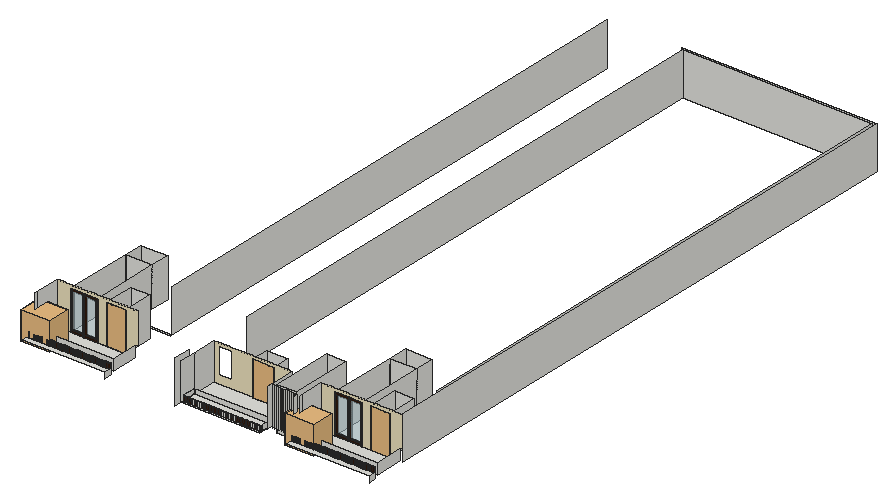
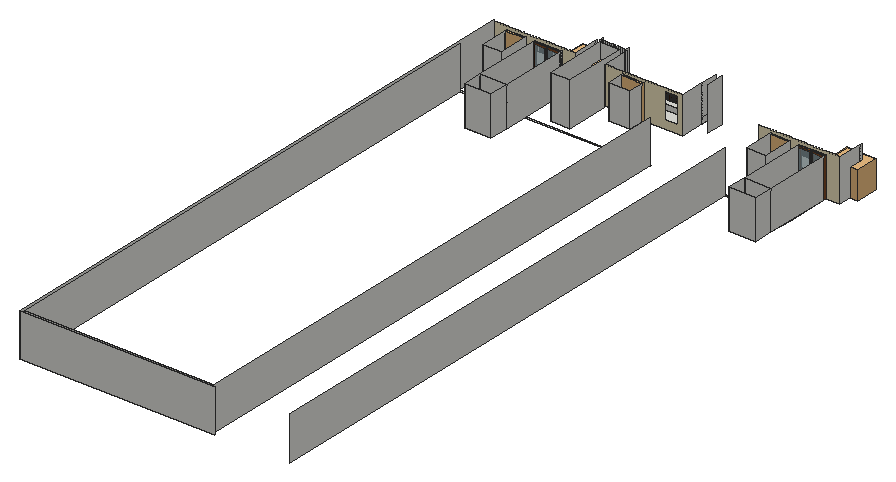
# SketchUp Ruby script. Lengths in inches.
U = 1.inch
M = Sketchup.active_model
def pt(a) = Geom::Point3d.new(a.map { |v| v * U })
def face(e, loops, mat)
  f = e.add_face(loops[0].map { |a| pt(a) })
  loops[1..].each { |l| e.add_face(l.map { |a| pt(a) }).erase! }
  f.material = f.back_material = mat if mat
  f
end
# faces: each face lists its corners as indices into pts; further lists are holes
def faces(e, pts, list, mat = nil) = list.each { |f| face(e, (f[0].is_a?(Array) ? f : [f]).map { |l| l.map { |i| pts[i] } }, mat) }
# xy, xz, yz: faces in a plane at the given z, y or x. An outline is a flat list of corners, or four numbers for a rectangle; further outlines are holes
def ring(l) = l.size == 4 ? [[l[0], l[1]], [l[2], l[1]], [l[2], l[3]], [l[0], l[3]]] : l.each_slice(2).to_a
def flat(e, list, mat, &to3) = list.each { |f| face(e, (f[0].is_a?(Array) ? f : [f]).map { |l| ring(l).map { |u, v| to3.(u, v) } }, mat) }
def xy(e, z, list, mat = nil) = flat(e, list, mat) { |x, y| [x, y, z] }
def xz(e, y, list, mat = nil) = flat(e, list, mat) { |x, z| [x, y, z] }
def yz(e, x, list, mat = nil) = flat(e, list, mat) { |y, z| [x, y, z] }
def lines(e, pts, list) = list.each { |a, b| e.add_line(pt(pts[a]), pt(pts[b])) }
# prism: a flat outline (further loops are holes) pulled along v
def prism(e, loops, v, mat = nil)
  f = face(e, loops, mat); d = Geom::Vector3d.new(v.map { |x| x * U })
  f.pushpull(f.normal.samedirection?(d) ? d.length : -d.length)
end
def box(e, o, s, mat = nil) = prism(e, [[o, [o[0] + s[0], o[1], o[2]], [o[0] + s[0], o[1] + s[1], o[2]], [o[0], o[1] + s[1], o[2]]]], [0, 0, s[2]], mat)
def at(x, y, z, deg = 0) = Geom::Transformation.translation(pt([x, y, z])) * Geom::Transformation.rotation(ORIGIN, Z_AXIS, deg.degrees)
def axes(o, x, y, z) = Geom::Transformation.new([*x, 0, *y, 0, *z, 0, *pt(o).to_a, 1])
def part(name) = M.definitions.add(name)
# library, detail: a bought-in or finely detailed component or shape, given as its bounding box
def library(name, o, s) = part(name).tap { |d| box(d.entities, o, s) }
def detail(e, o, s) = box(e.add_group.entities, o, s)
def put(e, d, t, mat = nil) = e.add_instance(d, t).tap { |i| i.material = mat if mat }
def group(e, t, mat = nil) = e.add_group.tap { |g| g.transformation = t; g.material = mat if mat }.entities
root = M.entities
M.materials.add("[Color D01]").color = [237, 225, 189]
M.materials.add("[Translucent Glass Safety]").color = [204, 235, 244]
M.materials["[Translucent Glass Safety]"].alpha = 0.5
M.materials.add("[Wood Veneer 01]").color = [51, 28, 15]
M.materials.add("[Wood Veneer 01]1").color = [120, 70, 37]
c1 = library("Round Planter with Plant",[-35.48,-39.77,0],[80.62,63.55,77.875])
c2 = part("Component\#1")
xy(c2.entities,0,[[0,0,6,48]],"[Wood Veneer 01]1")
xy(c2.entities,4,[[0,4,1.8125,44],[1.8125,4,6,44]])
xy(c2.entities,80,[[0,4,1.8125,44],[1.8125,4,6,44]])
xy(c2.entities,84,[[0,0,6,48]],"[Wood Veneer 01]1")
xz(c2.entities,0,[[0,0,6,84]],"[Wood Veneer 01]1")
xz(c2.entities,4,[[0,4,1.8125,80],[1.8125,4,6,80]])
xz(c2.entities,44,[[0,4,1.8125,80],[1.8125,4,6,80]])
xz(c2.entities,48,[[0,0,6,84]],"[Wood Veneer 01]1")
yz(c2.entities,0,[[[0,0,48,84],[4,4,44,80]]],"[Wood Veneer 01]1")
yz(c2.entities,1.8125,[[4,4,44,80]],"[Translucent Glass Safety]")
yz(c2.entities,6,[[[0,0,48,84],[4,4,44,80]]],"[Wood Veneer 01]")
c3 = part("Group\#3")
put(c3.entities,c2,at(0,0,0),"[Wood Veneer 01]")
g1 = group(c3.entities,at(0,48,0),"[Wood Veneer 01]")
xy(g1,0,[[0,0,6,48]],"[Wood Veneer 01]1")
xy(g1,4,[[0,4,1.8125,44],[1.8125,4,6,44]])
xy(g1,80,[[0,4,1.8125,44],[1.8125,4,6,44]])
xy(g1,84,[[0,0,6,48]],"[Wood Veneer 01]1")
xz(g1,0,[[0,0,6,84]],"[Wood Veneer 01]1")
xz(g1,4,[[0,4,1.8125,80],[1.8125,4,6,80]])
xz(g1,44,[[0,4,1.8125,80],[1.8125,4,6,80]])
xz(g1,48,[[0,0,6,84]],"[Wood Veneer 01]1")
yz(g1,0,[[[0,0,48,84],[4,4,44,80]]],"[Wood Veneer 01]1")
yz(g1,1.8125,[[4,4,44,80]],"[Translucent Glass Safety]")
yz(g1,6,[[[0,0,48,84],[4,4,44,80]]],"[Wood Veneer 01]")
c4 = library("元件\#5",[-4.39,0,0],[5.37,35.83,90.55])
xy(root,386.6875,[[1130.14,286.21,1348.32,361.27],[1863.7,286.21,2081.89,361.27],[1169.05,361.27,1243.3,483.79],[1268.48,361.27,1321.23,445.08],[1902.61,361.27,1976.86,483.79],
  [2002.05,361.27,2054.8,445.08],[1169.05,483.79,1243.3,551.2],[1243.3,483.79,1348.32,488.08],[1557.49,483.79,1902.61,488.08],[1902.61,483.79,1976.86,551.2],
  [1976.86,483.79,2081.89,488.08],[1169.05,551.2,1243.3,604.39],[1902.61,551.2,1976.86,604.39]])
xy(root,402.5,[[1567.3,255.92,1776.61,293.45],[1567.3,293.45,1782.56,293.45,1782.56,361.27,1733.6,361.27,1733.6,408.14,1674.93,408.14,1674.93,361.27,1567.3,361.27]])
xy(root,403.1875,[[1127.51,246.64,1355.5625,246.64,1355.5625,266.43,1132.28,266.43,1132.28,263.8,1127.51,263.8],[1567.3,246.64,1785.93,246.64,1785.93,286.21,1782.8,286.21,1782.8,253.61,1567.3,253.61],[1861.07,246.64,2089.125,246.64,2089.125,266.43,1865.84,266.43,1865.84,263.8,1861.07,263.8],[1567.3,253.61,1776.61,255.92]])
xz(root,253.61,[[1570.91,403.1875,1572.05,416.75],[1575.66,403.1875,1576.8,416.75],[1580.41,403.1875,1581.55,416.75],[1585.16,403.1875,1586.3,416.75],[1589.91,403.1875,1591.05,416.75],
  [1594.66,403.1875,1595.8,416.75],[1599.41,403.1875,1600.55,416.75],[1604.16,403.1875,1605.3,416.75],[1608.91,403.1875,1610.05,416.75],[1613.66,403.1875,1614.8,416.75],
  [1618.41,403.1875,1619.55,416.75],[1623.16,403.1875,1624.3,416.75],[1627.91,403.1875,1629.05,416.75],[1632.66,403.1875,1633.8,416.75],[1637.41,403.1875,1638.55,416.75],
  [1642.16,403.1875,1643.3,416.75],[1646.91,403.1875,1648.05,416.75],[1651.66,403.1875,1652.8,416.75],[1656.41,403.1875,1657.55,416.75],[1661.16,403.1875,1662.3,416.75],
  [1665.91,403.1875,1667.05,416.75],[1670.66,403.1875,1671.8,416.75],[1675.41,403.1875,1676.55,416.75],[1680.16,403.1875,1681.3,416.75],[1684.91,403.1875,1686.05,416.75],
  [1689.66,403.1875,1690.8,416.75],[1694.41,403.1875,1695.55,416.75],[1699.16,403.1875,1700.3,416.75],[1703.91,403.1875,1705.05,416.75],[1708.66,403.1875,1709.8,416.75],
  [1713.41,403.1875,1714.55,416.75],[1718.16,403.1875,1719.3,416.75],[1722.91,403.1875,1724.05,416.75],[1727.66,403.1875,1728.8,416.75],[1732.41,403.1875,1733.55,416.75],
  [1737.16,403.1875,1738.3,416.75],[1741.91,403.1875,1743.05,416.75],[1746.66,403.1875,1747.8,416.75],[1751.41,403.1875,1752.55,416.75],[1756.16,403.1875,1757.3,416.75],
  [1760.91,403.1875,1762.05,416.75],[1765.66,403.1875,1766.8,416.75],[1770.41,403.1875,1771.55,416.75],[1775.16,403.1875,1776.3,416.75],[1779.91,403.1875,1781.05,416.75]])
xz(root,253.61,[[1567.3,403.1875,1570.91,416.75],[1572.05,403.1875,1575.66,416.75],[1576.8,403.1875,1580.41,416.75],[1581.55,403.1875,1585.16,416.75],[1586.3,403.1875,1589.91,416.75],
  [1591.05,403.1875,1594.66,416.75],[1595.8,403.1875,1599.41,416.75],[1600.55,403.1875,1604.16,416.75],[1605.3,403.1875,1608.91,416.75],[1610.05,403.1875,1613.66,416.75],
  [1614.8,403.1875,1618.41,416.75],[1619.55,403.1875,1623.16,416.75],[1624.3,403.1875,1627.91,416.75],[1629.05,403.1875,1632.66,416.75],[1633.8,403.1875,1637.41,416.75],
  [1638.55,403.1875,1642.16,416.75],[1643.3,403.1875,1646.91,416.75],[1648.05,403.1875,1651.66,416.75],[1652.8,403.1875,1656.41,416.75],[1657.55,403.1875,1661.16,416.75],
  [1662.3,403.1875,1665.91,416.75],[1667.05,403.1875,1670.66,416.75],[1671.8,403.1875,1675.41,416.75],[1676.55,403.1875,1680.16,416.75],[1681.3,403.1875,1684.91,416.75],
  [1686.05,403.1875,1689.66,416.75],[1690.8,403.1875,1694.41,416.75],[1695.55,403.1875,1699.16,416.75],[1700.3,403.1875,1703.91,416.75],[1705.05,403.1875,1708.66,416.75],
  [1709.8,403.1875,1713.41,416.75],[1714.55,403.1875,1718.16,416.75],[1719.3,403.1875,1722.91,416.75],[1724.05,403.1875,1727.66,416.75],[1728.8,403.1875,1732.41,416.75],
  [1733.55,403.1875,1737.16,416.75],[1738.3,403.1875,1741.91,416.75],[1743.05,403.1875,1746.66,416.75],[1747.8,403.1875,1751.41,416.75],[1752.55,403.1875,1756.16,416.75],
  [1757.3,403.1875,1760.91,416.75],[1762.05,403.1875,1765.66,416.75],[1766.8,403.1875,1770.41,416.75],[1771.55,403.1875,1775.16,416.75],[1776.3,403.1875,1779.91,416.75],
  [1781.05,403.1875,1782.8,416.75],[1782.8,403.1875,1784.66,416.75]],"[Wood Veneer 01]")
xz(root,255.92,[[1567.3,402.5,1776.61,403.1875]])
xz(root,263.8,[[1133.51,403.1875,1138.28,416.75],[1139.51,403.1875,1144.28,416.75],[1145.51,403.1875,1150.28,416.75],[1151.51,403.1875,1156.28,416.75],[1157.51,403.1875,1162.28,416.75],
  [1163.51,403.1875,1168.28,416.75],[1169.51,403.1875,1174.28,416.75],[1175.51,403.1875,1180.28,416.75],[1181.51,403.1875,1186.28,416.75],[1187.51,403.1875,1192.28,416.75],
  [1193.51,403.1875,1198.28,416.75],[1199.51,403.1875,1204.28,416.75],[1205.51,403.1875,1210.28,416.75],[1211.51,403.1875,1216.28,416.75],[1217.51,403.1875,1222.28,416.75],
  [1223.51,403.1875,1228.28,416.75],[1229.51,403.1875,1234.28,416.75],[1235.51,403.1875,1240.28,416.75],[1241.51,403.1875,1246.28,416.75],[1247.51,403.1875,1252.28,416.75],
  [1253.51,403.1875,1258.28,416.75],[1259.51,403.1875,1264.28,416.75],[1265.51,403.1875,1270.28,416.75],[1271.51,403.1875,1276.28,416.75],[1277.51,403.1875,1282.28,416.75],
  [1283.51,403.1875,1288.28,416.75],[1289.51,403.1875,1294.28,416.75],[1295.51,403.1875,1300.28,416.75],[1301.51,403.1875,1306.28,416.75],[1307.51,403.1875,1312.28,416.75],
  [1313.51,403.1875,1318.28,416.75],[1319.51,403.1875,1324.28,416.75],[1325.51,403.1875,1330.28,416.75],[1331.51,403.1875,1336.28,416.75],[1337.51,403.1875,1342.28,416.75],
  [1343.51,403.1875,1348.28,416.75],[1349.51,403.1875,1354.28,416.75],[1861.07,403.1875,1865.84,416.75],[1867.07,403.1875,1871.84,416.75],[1873.07,403.1875,1877.84,416.75],
  [1879.07,403.1875,1883.84,416.75],[1885.07,403.1875,1889.84,416.75],[1891.07,403.1875,1895.84,416.75],[1897.07,403.1875,1901.84,416.75],[1903.07,403.1875,1907.84,416.75],
  [1909.07,403.1875,1913.84,416.75],[1915.07,403.1875,1919.84,416.75],[1921.07,403.1875,1925.84,416.75],[1927.07,403.1875,1931.84,416.75],[1933.07,403.1875,1937.84,416.75],
  [1939.07,403.1875,1943.84,416.75],[1945.07,403.1875,1949.84,416.75],[1951.07,403.1875,1955.84,416.75],[1957.07,403.1875,1961.84,416.75],[1963.07,403.1875,1967.84,416.75],
  [1969.07,403.1875,1973.84,416.75],[1975.07,403.1875,1979.84,416.75],[1981.07,403.1875,1985.84,416.75],[1987.07,403.1875,1991.84,416.75],[1993.07,403.1875,1997.84,416.75],
  [1999.07,403.1875,2003.84,416.75],[2005.07,403.1875,2009.84,416.75],[2011.07,403.1875,2015.84,416.75],[2017.07,403.1875,2021.84,416.75],[2023.07,403.1875,2027.84,416.75],
  [2029.07,403.1875,2033.84,416.75],[2035.07,403.1875,2039.84,416.75],[2041.07,403.1875,2045.84,416.75],[2047.07,403.1875,2051.84,416.75],[2053.07,403.1875,2057.84,416.75],
  [2059.07,403.1875,2063.84,416.75],[2065.07,403.1875,2069.84,416.75],[2071.07,403.1875,2075.84,416.75],[2077.07,403.1875,2081.84,416.75],[2083.07,403.1875,2087.84,416.75]],"[Wood Veneer 01]")
xz(root,266.43,[[1132.28,403.1875,1138.28,416.75],[1138.28,403.1875,1144.28,416.75],[1144.28,403.1875,1150.28,416.75],[1150.28,403.1875,1156.28,416.75],[1156.28,403.1875,1162.28,416.75],
  [1162.28,403.1875,1168.28,416.75],[1168.28,403.1875,1174.28,416.75],[1174.28,403.1875,1180.28,416.75],[1180.28,403.1875,1186.28,416.75],[1186.28,403.1875,1192.28,416.75],
  [1192.28,403.1875,1198.28,416.75],[1198.28,403.1875,1204.28,416.75],[1204.28,403.1875,1210.28,416.75],[1210.28,403.1875,1216.28,416.75],[1216.28,403.1875,1222.28,416.75],
  [1222.28,403.1875,1228.28,416.75],[1228.28,403.1875,1234.28,416.75],[1234.28,403.1875,1240.28,416.75],[1240.28,403.1875,1246.28,416.75],[1246.28,403.1875,1252.28,416.75],
  [1252.28,403.1875,1258.28,416.75],[1258.28,403.1875,1264.28,416.75],[1264.28,403.1875,1270.28,416.75],[1270.28,403.1875,1276.28,416.75],[1276.28,403.1875,1282.28,416.75],
  [1282.28,403.1875,1288.28,416.75],[1288.28,403.1875,1294.28,416.75],[1294.28,403.1875,1300.28,416.75],[1300.28,403.1875,1306.28,416.75],[1306.28,403.1875,1312.28,416.75],
  [1312.28,403.1875,1318.28,416.75],[1318.28,403.1875,1324.28,416.75],[1324.28,403.1875,1330.28,416.75],[1330.28,403.1875,1336.28,416.75],[1336.28,403.1875,1342.28,416.75],
  [1342.28,403.1875,1348.28,416.75],[1348.28,403.1875,1348.32,416.75],[1348.32,403.1875,1354.28,416.75],[1354.28,403.1875,1355.5625,416.75],[1865.84,403.1875,1871.84,416.75],
  [1871.84,403.1875,1877.84,416.75],[1877.84,403.1875,1883.84,416.75],[1883.84,403.1875,1889.84,416.75],[1889.84,403.1875,1895.84,416.75],[1895.84,403.1875,1901.84,416.75],
  [1901.84,403.1875,1907.84,416.75],[1907.84,403.1875,1913.84,416.75],[1913.84,403.1875,1919.84,416.75],[1919.84,403.1875,1925.84,416.75],[1925.84,403.1875,1931.84,416.75],
  [1931.84,403.1875,1937.84,416.75],[1937.84,403.1875,1943.84,416.75],[1943.84,403.1875,1949.84,416.75],[1949.84,403.1875,1955.84,416.75],[1955.84,403.1875,1961.84,416.75],
  [1961.84,403.1875,1967.84,416.75],[1967.84,403.1875,1973.84,416.75],[1973.84,403.1875,1979.84,416.75],[1979.84,403.1875,1985.84,416.75],[1985.84,403.1875,1991.84,416.75],
  [1991.84,403.1875,1997.84,416.75],[1997.84,403.1875,2003.84,416.75],[2003.84,403.1875,2009.84,416.75],[2009.84,403.1875,2015.84,416.75],[2015.84,403.1875,2021.84,416.75],
  [2021.84,403.1875,2027.84,416.75],[2027.84,403.1875,2033.84,416.75],[2033.84,403.1875,2039.84,416.75],[2039.84,403.1875,2045.84,416.75],[2045.84,403.1875,2051.84,416.75],
  [2051.84,403.1875,2057.84,416.75],[2057.84,403.1875,2063.84,416.75],[2063.84,403.1875,2069.84,416.75],[2069.84,403.1875,2075.84,416.75],[2075.84,403.1875,2081.84,416.75],
  [2081.84,403.1875,2081.89,416.75],[2081.89,403.1875,2087.84,416.75],[2087.84,403.1875,2089.125,416.75]])
xz(root,286.21,[[1130.14,386.6875,1348.32,416.75],[1861.07,386.6875,1863.7,403.1875],[1863.7,386.6875,2081.89,416.75],[1782.8,403.1875,1785.93,403.1875,1785.93,505.3125,1782.56,505.3125,1782.56,409.375,1782.8,409.375],[1861.07,403.1875,1863.7,416.75]])
xz(root,293.45,[[1795.15,386.6875,1849.87,506.6875],[1567.3,402.5,1567.3,416.75,1782.56,416.75,1782.56,409.375,1776.61,409.375,1776.61,402.5],[1776.61,402.5,1782.56,409.375]])
xz(root,361.27,[[1130.14,386.6875,1169.05,386.6875,1169.05,495.625,1243.3,495.625,1243.3,386.6875,1268.48,386.6875,1268.48,495.6875,1321.23,495.6875,1321.23,386.6875,1348.32,386.6875,1348.32,418.9375,1355.5625,418.9375,1355.5625,505.3125,1349.34,505.3125,1349.34,504,1342.64,504,1342.64,505.3125,1340.84,505.3125,1340.84,504,1334.14,504,1334.14,505.3125,1332.34,505.3125,1332.34,504,1325.64,504,1325.64,505.3125,1323.84,505.3125,1323.84,504,1317.14,504,1317.14,505.3125,1315.34,505.3125,1315.34,504,1308.64,504,1308.64,505.3125,1306.84,505.3125,1306.84,504,1300.14,504,1300.14,505.3125,1298.34,505.3125,1298.34,504,1291.64,504,1291.64,505.3125,1289.84,505.3125,1289.84,504,1283.14,504,1283.14,505.3125,1281.34,505.3125,1281.34,504,1274.64,504,1274.64,505.3125,1272.84,505.3125,1272.84,504,1266.14,504,1266.14,505.3125,1264.34,505.3125,1264.34,504,1257.64,504,1257.64,505.3125,1255.84,505.3125,1255.84,504,1249.14,504,1249.14,505.3125,1247.34,505.3125,1247.34,504,1240.64,504,1240.64,505.3125,1238.84,505.3125,1238.84,504,1232.14,504,1232.14,505.3125,1230.34,505.3125,1230.34,504,1223.64,504,1223.64,505.3125,1221.84,505.3125,1221.84,504,1215.14,504,1215.14,505.3125,1213.34,505.3125,1213.34,504,1206.64,504,1206.64,505.3125,1204.84,505.3125,1204.84,504,1198.14,504,1198.14,505.3125,1196.34,505.3125,1196.34,504,1189.64,504,1189.64,505.3125,1187.84,505.3125,1187.84,504,1181.14,504,1181.14,505.3125,1179.34,505.3125,1179.34,504,1172.64,504,1172.64,505.3125,1170.84,505.3125,1170.84,504,1164.14,504,1164.14,505.3125,1162.34,505.3125,1162.34,504,1155.64,504,1155.64,505.3125,1153.84,505.3125,1153.84,504,1147.14,504,1147.14,505.3125,1145.34,505.3125,1145.34,504,1138.64,504,1138.64,505.3125,1136.84,505.3125,1136.84,504,1130.14,504],[1863.7,386.6875,1902.61,386.6875,1902.61,495.625,1976.86,495.625,1976.86,386.6875,2002.05,386.6875,2002.05,495.6875,2054.8,495.6875,2054.8,386.6875,2081.89,386.6875,2081.89,418.9375,2089.125,418.9375,2089.125,505.3125,2082.9,505.3125,2082.9,504,2076.2,504,2076.2,505.3125,2074.4,505.3125,2074.4,504,2067.7,504,2067.7,505.3125,2065.9,505.3125,2065.9,504,2059.2,504,2059.2,505.3125,2057.4,505.3125,2057.4,504,2050.7,504,2050.7,505.3125,2048.9,505.3125,2048.9,504,2042.2,504,2042.2,505.3125,2040.4,505.3125,2040.4,504,2033.7,504,2033.7,505.3125,2031.9,505.3125,2031.9,504,2025.2,504,2025.2,505.3125,2023.4,505.3125,2023.4,504,2016.7,504,2016.7,505.3125,2014.9,505.3125,2014.9,504,2008.2,504,2008.2,505.3125,2006.4,505.3125,2006.4,504,1999.7,504,1999.7,505.3125,1997.9,505.3125,1997.9,504,1991.2,504,1991.2,505.3125,1989.4,505.3125,1989.4,504,1982.7,504,1982.7,505.3125,1980.9,505.3125,1980.9,504,1974.2,504,1974.2,505.3125,1972.4,505.3125,1972.4,504,1965.7,504,1965.7,505.3125,1963.9,505.3125,1963.9,504,1957.2,504,1957.2,505.3125,1955.4,505.3125,1955.4,504,1948.7,504,1948.7,505.3125,1946.9,505.3125,1946.9,504,1940.2,504,1940.2,505.3125,1938.4,505.3125,1938.4,504,1931.7,504,1931.7,505.3125,1929.9,505.3125,1929.9,504,1923.2,504,1923.2,505.3125,1921.4,505.3125,1921.4,504,1914.7,504,1914.7,505.3125,1912.9,505.3125,1912.9,504,1906.2,504,1906.2,505.3125,1904.4,505.3125,1904.4,504,1897.7,504,1897.7,505.3125,1895.9,505.3125,1895.9,504,1889.2,504,1889.2,505.3125,1887.4,505.3125,1887.4,504,1880.7,504,1880.7,505.3125,1878.9,505.3125,1878.9,504,1872.2,504,1872.2,505.3125,1870.4,505.3125,1870.4,504,1863.7,504],[[1567.3,402.5,1674.93,402.5,1674.93,497.42,1733.6,497.42,1733.6,402.5,1782.56,402.5,1782.56,503.875,1777.07,503.875,1777.07,505.3125,1774.56,505.3125,1774.56,503.875,1769.07,503.875,1769.07,505.3125,1766.56,505.3125,1766.56,503.875,1761.07,503.875,1761.07,505.3125,1758.56,505.3125,1758.56,503.875,1753.07,503.875,1753.07,505.3125,1750.56,505.3125,1750.56,503.875,1745.07,503.875,1745.07,505.3125,1742.56,505.3125,1742.56,503.875,1737.07,503.875,1737.07,505.3125,1734.56,505.3125,1734.56,503.875,1729.07,503.875,1729.07,505.3125,1726.56,505.3125,1726.56,503.875,1721.07,503.875,1721.07,505.3125,1718.56,505.3125,1718.56,504,1713.07,504,1713.07,505.3125,1710.56,505.3125,1710.56,504,1705.07,504,1705.07,505.3125,1702.56,505.3125,1702.56,504,1697.07,504,1697.07,505.3125,1694.56,505.3125,1694.56,504,1689.07,504,1689.07,505.3125,1686.56,505.3125,1686.56,504,1681.07,504,1681.07,505.3125,1678.56,505.3125,1678.56,504,1673.07,504,1673.07,505.3125,1670.56,505.3125,1670.56,504,1665.07,504,1665.07,505.3125,1662.56,505.3125,1662.56,504,1657.07,504,1657.07,505.3125,1654.56,505.3125,1654.56,504,1649.07,504,1649.07,505.3125,1646.56,505.3125,1646.56,504,1641.07,504,1641.07,505.3125,1638.56,505.3125,1638.56,504,1633.07,504,1633.07,505.3125,1630.56,505.3125,1630.56,504,1625.07,504,1625.07,505.3125,1622.56,505.3125,1622.56,504,1617.07,504,1617.07,505.3125,1614.56,505.3125,1614.56,504,1609.07,504,1609.07,505.3125,1606.56,505.3125,1606.56,504,1601.07,504,1601.07,505.3125,1598.56,505.3125,1598.56,504,1593.07,504,1593.07,505.3125,1590.56,505.3125,1590.56,504,1585.07,504,1585.07,505.3125,1582.56,505.3125,1582.56,504,1577.07,504,1577.07,505.3125,1567.3,505.3125],[1579.05,425.31,1616.36,497.43]]],"[Color D01]")
xz(root,408.14,[[1674.93,402.5,1733.6,497.42]])
xz(root,445.08,[[1268.48,386.6875,1321.23,495.6875],[2002.05,386.6875,2054.8,495.6875]])
xz(root,465.02,[[1795.15,386.6875,1849.87,506.6875]])
xz(root,551.2,[[1169.05,386.6875,1243.3,495.625],[1902.61,386.6875,1976.86,495.625]])
xz(root,604.39,[[1169.05,386.6875,1243.3,495.625],[1902.61,386.6875,1976.86,495.625]])
xz(root,1996.66,[[1557.49,386.6875,2081.89,506.6875]])
xz(root,2003.89,[[1550.25,386.6875,2089.125,506.6875]])
yz(root,1130.14,[[286.21,386.6875,293.45,504],[293.45,386.6875,361.27,504]])
yz(root,1132.28,[[263.8,403.1875,266.43,416.75]])
yz(root,1138.28,[[263.8,403.1875,266.43,416.75]])
yz(root,1144.28,[[263.8,403.1875,266.43,416.75]])
yz(root,1150.28,[[263.8,403.1875,266.43,416.75]])
yz(root,1156.28,[[263.8,403.1875,266.43,416.75]])
yz(root,1162.28,[[263.8,403.1875,266.43,416.75]])
yz(root,1168.28,[[263.8,403.1875,266.43,416.75]])
yz(root,1169.05,[[361.27,386.6875,551.2,495.625],[551.2,386.6875,604.39,495.625]])
yz(root,1174.28,[[263.8,403.1875,266.43,416.75]])
yz(root,1180.28,[[263.8,403.1875,266.43,416.75]])
yz(root,1186.28,[[263.8,403.1875,266.43,416.75]])
yz(root,1192.28,[[263.8,403.1875,266.43,416.75]])
yz(root,1198.28,[[263.8,403.1875,266.43,416.75]])
yz(root,1204.28,[[263.8,403.1875,266.43,416.75]])
yz(root,1210.28,[[263.8,403.1875,266.43,416.75]])
yz(root,1216.28,[[263.8,403.1875,266.43,416.75]])
yz(root,1222.28,[[263.8,403.1875,266.43,416.75]])
yz(root,1228.28,[[263.8,403.1875,266.43,416.75]])
yz(root,1234.28,[[263.8,403.1875,266.43,416.75]])
yz(root,1240.28,[[263.8,403.1875,266.43,416.75]])
yz(root,1243.3,[[361.27,386.6875,551.2,495.625],[551.2,386.6875,604.39,495.625]])
yz(root,1246.28,[[263.8,403.1875,266.43,416.75]])
yz(root,1252.28,[[263.8,403.1875,266.43,416.75]])
yz(root,1258.28,[[263.8,403.1875,266.43,416.75]])
yz(root,1264.28,[[263.8,403.1875,266.43,416.75]])
yz(root,1268.48,[[361.27,386.6875,445.08,495.6875]])
yz(root,1270.28,[[263.8,403.1875,266.43,416.75]])
yz(root,1276.28,[[263.8,403.1875,266.43,416.75]])
yz(root,1282.28,[[263.8,403.1875,266.43,416.75]])
yz(root,1288.28,[[263.8,403.1875,266.43,416.75]])
yz(root,1294.28,[[263.8,403.1875,266.43,416.75]])
yz(root,1300.28,[[263.8,403.1875,266.43,416.75]])
yz(root,1306.28,[[263.8,403.1875,266.43,416.75]])
yz(root,1312.28,[[263.8,403.1875,266.43,416.75]])
yz(root,1318.28,[[263.8,403.1875,266.43,416.75]])
yz(root,1321.23,[[361.27,386.6875,445.08,495.6875]])
yz(root,1324.28,[[263.8,403.1875,266.43,416.75]])
yz(root,1330.28,[[263.8,403.1875,266.43,416.75]])
yz(root,1336.28,[[263.8,403.1875,266.43,416.75]])
yz(root,1342.28,[[263.8,403.1875,266.43,416.75]])
yz(root,1348.32,[[286.21,386.6875,361.27,416.75],[488.08,386.6875,1996.66,506.6875]])
yz(root,1355.5625,[[246.64,386.6875,266.43,403.1875]])
yz(root,1550.25,[[246.64,386.6875,293.46,506.6875]])
yz(root,1557.49,[[488.08,386.6875,1996.66,506.6875]])
yz(root,1567.3,[[255.92,402.5,293.45,403.1875],[293.45,402.5,293.46,403.1875],[293.46,402.5,361.27,505.3125],[246.64,403.1875,253.61,403.1875,253.61,416.75,253.3,416.75,253.3,418.9375,293.45,418.9375,293.45,403.1875,293.46,403.1875,293.46,505.3125,246.64,505.3125],[253.61,403.1875,293.45,416.75]])
yz(root,1674.93,[[361.27,402.5,408.14,497.42]])
yz(root,1733.6,[[361.27,402.5,408.14,497.42]])
yz(root,1782.56,[[293.45,402.5,361.27,503.875]])
yz(root,1782.8,[[253.61,403.1875,286.21,403.1875,286.21,409.375,293.45,409.375,293.45,416.75,253.61,416.75]])
yz(root,1785.93,[[271.96,403.1875,286.21,506.6875]])
yz(root,1791.93,[[282.52,403.1875,286.21,506.6875]])
yz(root,1795.15,[[293.45,386.6875,465.02,506.6875]])
yz(root,1797.93,[[282.52,403.1875,286.21,506.6875]])
yz(root,1803.93,[[282.52,403.1875,286.21,506.6875]])
yz(root,1809.93,[[282.52,403.1875,286.21,506.6875]])
yz(root,1815.93,[[283.46,403.1875,286.21,506.6875]])
yz(root,1821.93,[[283.46,403.1875,286.21,506.6875]])
yz(root,1827.93,[[283.46,403.1875,286.21,506.6875]])
yz(root,1833.93,[[283.46,403.1875,286.21,506.6875]])
yz(root,1839.93,[[283.46,403.1875,286.21,506.6875]])
yz(root,1845.93,[[283.46,403.1875,286.21,506.6875]])
yz(root,1849.87,[[293.45,386.6875,465.02,506.6875]])
yz(root,1851.93,[[283.46,403.1875,286.21,506.6875]])
yz(root,1857.25,[[272.89,403.1875,286.21,506.6875]])
yz(root,1861.07,[[263.8,403.1875,266.49,416.75]],"[Wood Veneer 01]")
yz(root,1863.7,[[286.21,386.6875,293.45,504],[293.45,386.6875,361.27,504]])
yz(root,1865.84,[[263.8,403.1875,266.43,416.75]])
yz(root,1871.84,[[263.8,403.1875,266.43,416.75]])
yz(root,1877.84,[[263.8,403.1875,266.43,416.75]])
yz(root,1883.84,[[263.8,403.1875,266.43,416.75]])
yz(root,1889.84,[[263.8,403.1875,266.43,416.75]])
yz(root,1895.84,[[263.8,403.1875,266.43,416.75]])
yz(root,1901.84,[[263.8,403.1875,266.43,416.75]])
yz(root,1902.61,[[361.27,386.6875,551.2,495.625],[551.2,386.6875,604.39,495.625]])
yz(root,1907.84,[[263.8,403.1875,266.43,416.75]])
yz(root,1913.84,[[263.8,403.1875,266.43,416.75]])
yz(root,1919.84,[[263.8,403.1875,266.43,416.75]])
yz(root,1925.84,[[263.8,403.1875,266.43,416.75]])
yz(root,1931.84,[[263.8,403.1875,266.43,416.75]])
yz(root,1937.84,[[263.8,403.1875,266.43,416.75]])
yz(root,1943.84,[[263.8,403.1875,266.43,416.75]])
yz(root,1949.84,[[263.8,403.1875,266.43,416.75]])
yz(root,1955.84,[[263.8,403.1875,266.43,416.75]])
yz(root,1961.84,[[263.8,403.1875,266.43,416.75]])
yz(root,1967.84,[[263.8,403.1875,266.43,416.75]])
yz(root,1973.84,[[263.8,403.1875,266.43,416.75]])
yz(root,1976.86,[[361.27,386.6875,551.2,495.625],[551.2,386.6875,604.39,495.625]])
yz(root,1979.84,[[263.8,403.1875,266.43,416.75]])
yz(root,1985.84,[[263.8,403.1875,266.43,416.75]])
yz(root,1991.84,[[263.8,403.1875,266.43,416.75]])
yz(root,1997.84,[[263.8,403.1875,266.43,416.75]])
yz(root,2002.05,[[361.27,386.6875,445.08,495.6875]])
yz(root,2003.84,[[263.8,403.1875,266.43,416.75]])
yz(root,2009.84,[[263.8,403.1875,266.43,416.75]])
yz(root,2015.84,[[263.8,403.1875,266.43,416.75]])
yz(root,2021.84,[[263.8,403.1875,266.43,416.75]])
yz(root,2027.84,[[263.8,403.1875,266.43,416.75]])
yz(root,2033.84,[[263.8,403.1875,266.43,416.75]])
yz(root,2039.84,[[263.8,403.1875,266.43,416.75]])
yz(root,2045.84,[[263.8,403.1875,266.43,416.75]])
yz(root,2051.84,[[263.8,403.1875,266.43,416.75]])
yz(root,2054.8,[[361.27,386.6875,445.08,495.6875]])
yz(root,2057.84,[[263.8,403.1875,266.43,416.75]])
yz(root,2063.84,[[263.8,403.1875,266.43,416.75]])
yz(root,2069.84,[[263.8,403.1875,266.43,416.75]])
yz(root,2075.84,[[263.8,403.1875,266.43,416.75]])
yz(root,2081.89,[[286.21,386.6875,361.27,416.75],[488.08,386.6875,1996.66,506.6875]])
yz(root,2089.125,[[246.64,386.6875,266.43,403.1875],[361.27,386.6875,2003.89,506.6875]])
put(root,c1,at(1143.37,303,386.6875))
put(root,c3,axes([1169.05,367.27,386.6875],[0,-1,0],[0.77344,0,0],[0,0,1.29687]))
put(root,c4,axes([1269.02,362.12,386.6875],[0,-0.89,0],[1.45734,0,0],[0,0,1.20374]))
put(root,c4,axes([1674.93,361.64,402.5],[0,-1,0],[1.63746,0,0],[0,0,1.04827]))
put(root,c1,at(1876.93,303,386.6875))
put(root,c3,axes([1902.61,367.27,386.6875],[0,-1,0],[0.77344,0,0],[0,0,1.29687]))
put(root,c4,axes([2002.58,362.12,386.6875],[0,-0.89,0],[1.45734,0,0],[0,0,1.20374]))
